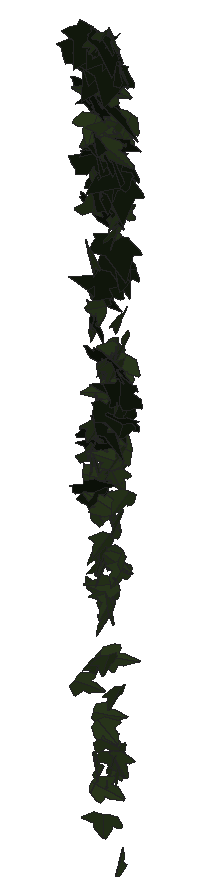
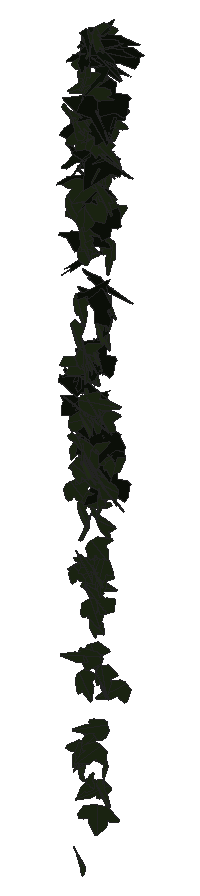
# SketchUp Ruby script. Lengths in inches.
U = 1.inch
M = Sketchup.active_model
def pt(a) = Geom::Point3d.new(a.map { |v| v * U })
def face(e, loops, mat)
  f = e.add_face(loops[0].map { |a| pt(a) })
  loops[1..].each { |l| e.add_face(l.map { |a| pt(a) }).erase! }
  f.material = f.back_material = mat if mat
  f
end
# faces: each face lists its corners as indices into pts; further lists are holes
def faces(e, pts, list, mat = nil) = list.each { |f| face(e, (f[0].is_a?(Array) ? f : [f]).map { |l| l.map { |i| pts[i] } }, mat) }
# xy, xz, yz: faces in a plane at the given z, y or x. An outline is a flat list of corners, or four numbers for a rectangle; further outlines are holes
def ring(l) = l.size == 4 ? [[l[0], l[1]], [l[2], l[1]], [l[2], l[3]], [l[0], l[3]]] : l.each_slice(2).to_a
def flat(e, list, mat, &to3) = list.each { |f| face(e, (f[0].is_a?(Array) ? f : [f]).map { |l| ring(l).map { |u, v| to3.(u, v) } }, mat) }
def xy(e, z, list, mat = nil) = flat(e, list, mat) { |x, y| [x, y, z] }
def xz(e, y, list, mat = nil) = flat(e, list, mat) { |x, z| [x, y, z] }
def yz(e, x, list, mat = nil) = flat(e, list, mat) { |y, z| [x, y, z] }
def lines(e, pts, list) = list.each { |a, b| e.add_line(pt(pts[a]), pt(pts[b])) }
# prism: a flat outline (further loops are holes) pulled along v
def prism(e, loops, v, mat = nil)
  f = face(e, loops, mat); d = Geom::Vector3d.new(v.map { |x| x * U })
  f.pushpull(f.normal.samedirection?(d) ? d.length : -d.length)
end
def box(e, o, s, mat = nil) = prism(e, [[o, [o[0] + s[0], o[1], o[2]], [o[0] + s[0], o[1] + s[1], o[2]], [o[0], o[1] + s[1], o[2]]]], [0, 0, s[2]], mat)
def at(x, y, z, deg = 0) = Geom::Transformation.translation(pt([x, y, z])) * Geom::Transformation.rotation(ORIGIN, Z_AXIS, deg.degrees)
def axes(o, x, y, z) = Geom::Transformation.new([*x, 0, *y, 0, *z, 0, *pt(o).to_a, 1])
def part(name) = M.definitions.add(name)
# library, detail: a bought-in or finely detailed component or shape, given as its bounding box
def library(name, o, s) = part(name).tap { |d| box(d.entities, o, s) }
def detail(e, o, s) = box(e.add_group.entities, o, s)
def put(e, d, t, mat = nil) = e.add_instance(d, t).tap { |i| i.material = mat if mat }
def group(e, t, mat = nil) = e.add_group.tap { |g| g.transformation = t; g.material = mat if mat }.entities
root = M.entities
M.materials.add("1026 AP 7946 SUNNY SIDE UP").color = [254, 231, 186]
M.materials.add("efeu1").color = [18, 25, 13]
M.materials.add("efeu2").color = [43, 57, 29]
c1 = part("ivyleaf_10")
p = [[0,0.5,-0.03],[-0.0625,2.02,-0.43],[-0.19,2.01,-0.46],[-0.54,1.05,-0.29],[-0.52,0.625,-0.18],[-0.83,0.76,-0.28],
  [-1.16,0.64,-0.33],[-1.15,0.33,-0.24],[-0.77,-0.39,0.02],[-0.3,-0.51,0.16],[0.04,-0.48,0.23],[-0.02,2.01,-0.4375],
  [-0.06,2.01,-0.43],[0.04,-0.49,0.23],[0.67,-0.49,0.14],[1.38,0.36,-0.2],[1.375,0.51,-0.24],[0.81,0.65,-0.19],
  [0.62,0.59,-0.15],[0.6,1.09,-0.28],[0.5,1.23,-0.31]]
faces(c1.entities,p,[[0,1,2,3,4,5,6,7,8,9,10],[11,12,0,13,14,15,16,17,18,19,20]],"efeu2")
c2 = part("ivyleaf_9")
p = [[1.54,2.16,1.25],[1.36,2.04,1.19],[-0.21,0.99,0.68],[-0.71,1.11,0.82],[-0.85,0.86,0.67],[-0.8,0.17,0.21],
  [-0.9,-0.01,0.1],[-0.67,-0.16,-0.02],[-0.08,-0.08,-0.05],[-0.03,-0.6,-0.4],[0.65,-0.88,-0.66],[0.83,-0.6,-0.49],
  [1.29,-0.42,-0.43],[1.8125,-0.07,-0.26],[1.21,0.44,0.15]]
faces(c2.entities,p,[[0,1,2,3,4,5,6,7,8,9,10,11,12,13,14]],"efeu1")
put(root,c1,axes([99.76,212.49,266.375],[0.08517,0.006,-0.24182],[-0.3837,0.00239,-0.05363],[0.00175,0.23145,0.01006]),"1026 AP 7946 SUNNY SIDE UP")
put(root,c2,axes([99.56,212.48,266.26],[0.11075,0.21792,-0.06124],[-0.02401,-0.05844,-0.24433],[-0.38297,0.06669,-0.00239]),"1026 AP 7946 SUNNY SIDE UP")
put(root,c1,axes([99.72,212.47,265.36],[-0.24212,0.01726,0.18054],[-0.27936,-0.06579,-0.14291],[0.06741,-0.21066,0.05618]),"1026 AP 7946 SUNNY SIDE UP")
put(root,c1,axes([99.48,212.33,258.37],[-0.13846,-0.2022,-0.00145],[-0.01239,0.00432,0.23331],[-0.34303,0.08146,-0.00784]),"1026 AP 7946 SUNNY SIDE UP")
put(root,c1,axes([99.56,212.56,264.48],[0.26352,-0.15611,-0.06063],[-0.07644,0.03216,-0.23505],[0.27014,0.16139,-0.00736]),"1026 AP 7946 SUNNY SIDE UP")
put(root,c2,axes([99.64,212.18,264.87],[-0.35667,0.10368,-0.02563],[-0.02399,0.02832,0.2504],[0.17957,0.20972,-0.01745]),"1026 AP 7946 SUNNY SIDE UP")
put(root,c1,axes([99.71,212.37,257.11],[0.16693,-0.00017,0.20356],[-0.29635,0.06729,0.10477],[-0.09333,-0.21398,0.03141]),"1026 AP 7946 SUNNY SIDE UP")
put(root,c1,axes([99.48,212.51,265.76],[0.28202,-0.15147,0.04086],[-0.02126,0.04548,0.23985],[-0.26515,-0.16475,0.02422]),"1026 AP 7946 SUNNY SIDE UP")
put(root,c1,axes([99.54,212.5625,253.86],[0.16321,-0.18368,0.02591],[0.0078,-0.02725,-0.21731],[0.29164,0.10352,-0.00869]),"1026 AP 7946 SUNNY SIDE UP")
put(root,c1,axes([99.53,212.38,263.85],[-0.18724,-0.24297,-0.03657],[-0.02415,-0.03047,0.27857],[-0.38504,0.12007,0.00031]),"1026 AP 7946 SUNNY SIDE UP")
put(root,c2,axes([99.78,212.16,257.77],[-0.28086,0.06421,-0.18603],[-0.25595,0.08041,0.19541],[0.16009,0.2412,-0.01395]),"1026 AP 7946 SUNNY SIDE UP")
put(root,c1,axes([99.53,212.47,256.28],[-0.02105,-0.17932,-0.11094],[0.06019,0.10297,-0.18267],[0.32252,-0.03092,0.02685]),"1026 AP 7946 SUNNY SIDE UP")
put(root,c2,axes([99.37,212.375,266.55],[0.42706,0.06153,-0.00314],[0.00359,-0.0254,-0.28585],[-0.09683,0.27043,-0.02446]),"1026 AP 7946 SUNNY SIDE UP")
put(root,c1,axes([99.41,212.1,253.51],[-0.09836,-0.09431,-0.18432],[0.22061,0.11389,-0.11205],[0.22802,-0.15087,0.0289]),"1026 AP 7946 SUNNY SIDE UP")
put(root,c2,axes([99.6,212.3125,267.66],[-0.3275,-0.14109,-0.01632],[0.03935,-0.00907,-0.25502],[0.23734,-0.19318,0.01976]),"1026 AP 7946 SUNNY SIDE UP")
put(root,c1,axes([99.44,212.47,258.59],[-0.21275,0.07912,-0.11622],[0.14396,-0.07034,-0.15918],[-0.17866,-0.15089,0.01012]),"1026 AP 7946 SUNNY SIDE UP")
put(root,c1,axes([99.58,212.42,253.91],[-0.03475,-0.21835,-0.02189],[0.00904,0.01953,-0.22594],[0.34465,-0.02253,0.00372]),"1026 AP 7946 SUNNY SIDE UP")
put(root,c1,axes([99.625,212.14,263.01],[-0.26211,0.17039,0.07833],[-0.10034,0.04237,-0.24482],[-0.27504,-0.17784,0.01467]),"1026 AP 7946 SUNNY SIDE UP")
put(root,c2,axes([99.36,212.2,267.45],[-0.07303,-0.10387,-0.24371],[0.1798,0.20019,-0.11714],[0.38252,-0.11393,0.00853]),"1026 AP 7946 SUNNY SIDE UP")
put(root,c1,axes([99.69,212.1,261.41],[0.08371,-0.05213,0.26704],[-0.23495,0.21258,0.07681],[-0.34355,-0.15808,0.01254]),"1026 AP 7946 SUNNY SIDE UP")
put(root,c1,axes([99.55,212.52,251.41],[0.15767,-0.17338,0.07724],[0.0386,-0.07332,-0.20623],[0.29513,0.10222,-0.01429]),"1026 AP 7946 SUNNY SIDE UP")
put(root,c1,axes([99.58,212.625,258.77],[-0.01506,-0.15587,0.15875],[0.03486,-0.15503,-0.16011],[0.34386,0.00889,0.02318]),"1026 AP 7946 SUNNY SIDE UP")
put(root,c2,axes([99.36,212.59,265.85],[0.21526,-0.15628,0.09252],[0.08295,-0.07417,-0.21632],[0.29333,0.13566,-0.00672]),"1026 AP 7946 SUNNY SIDE UP")
put(root,c1,axes([99.8,212.61,259.78],[-0.06157,0.02381,0.22766],[-0.2122,-0.18068,-0.00564],[0.27744,-0.13291,0.04621]),"1026 AP 7946 SUNNY SIDE UP")
put(root,c2,axes([99.35,212.51,263.73],[0.32534,-0.07202,-0.12624],[0.20214,0.00416,0.22186],[-0.09403,-0.24023,0.04016]),"1026 AP 7946 SUNNY SIDE UP")
put(root,c1,axes([99.47,212.37,258.27],[-0.04813,0.0255,0.22754],[0.22348,-0.16655,0.03794],[0.28582,0.13452,0.00866]),"1026 AP 7946 SUNNY SIDE UP")
put(root,c1,axes([99.64,212.45,257.75],[0.05416,-0.15376,-0.15025],[0.00352,0.14021,-0.16437],[0.35109,0.02231,0.02483]),"1026 AP 7946 SUNNY SIDE UP")
put(root,c1,axes([99.64,212.4375,256.05],[-0.04484,-0.20123,-0.04817],[0.01543,0.04467,-0.20909],[0.32407,-0.02997,0.00329]),"1026 AP 7946 SUNNY SIDE UP")
put(root,c2,axes([99.6,212.29,259.03],[0.21165,0.18417,-0.00479],[0.01282,-0.0134,-0.23784],[-0.3126,0.12415,-0.01299]),"1026 AP 7946 SUNNY SIDE UP")
put(root,c1,axes([99.64,212.43,261.38],[0.09194,-0.21347,0.04998],[0.00429,-0.05076,-0.22806],[0.34462,0.05758,-0.0105]),"1026 AP 7946 SUNNY SIDE UP")
put(root,c1,axes([99.6,212.3,265.82],[0.35179,0.08539,-0.03383],[-0.03769,-0.03161,-0.23939],[-0.15058,0.20741,-0.01911]),"1026 AP 7946 SUNNY SIDE UP")
put(root,c1,axes([99.58,212.41,259.63],[-0.07566,0.14133,-0.10499],[0.0339,-0.09828,-0.15975],[-0.29185,-0.04805,0.00866]),"1026 AP 7946 SUNNY SIDE UP")
put(root,c2,axes([99.73,212.31,258.75],[0.17736,0.15221,-0.12069],[-0.13961,-0.08201,-0.19783],[-0.29187,0.13172,0.02129]),"1026 AP 7946 SUNNY SIDE UP")
put(root,c1,axes([99.58,212.59,256.1875],[0.12198,-0.14491,0.14792],[0.10082,-0.12944,-0.17005],[0.30547,0.10059,-0.00294]),"1026 AP 7946 SUNNY SIDE UP")
put(root,c1,axes([99.77,212.29,264.79],[-0.33099,0.02229,0.07366],[-0.11999,-0.02094,-0.20837],[-0.02367,-0.20561,0.02628]),"1026 AP 7946 SUNNY SIDE UP")
put(root,c2,axes([99.59,212.38,265.09],[0.26162,0.1795,0.00575],[0.02563,-0.0089,-0.25151],[-0.28117,0.1662,-0.01757]),"1026 AP 7946 SUNNY SIDE UP")
put(root,c2,axes([99.93,212.28,262.27],[-0.22067,0.10407,0.14173],[-0.19513,0.06503,-0.17648],[-0.20641,-0.17274,0.01532]),"1026 AP 7946 SUNNY SIDE UP")
put(root,c1,axes([99.64,212.24,258.48],[-0.17778,0.20569,0.00456],[-0.01956,-0.00312,-0.24149],[-0.32288,-0.11307,0.01212]),"1026 AP 7946 SUNNY SIDE UP")
put(root,c2,axes([99.62,212.35,267.4],[-0.26915,-0.16923,-0.05648],[0.11001,0.00745,-0.24421],[0.27891,-0.16625,0.04182]),"1026 AP 7946 SUNNY SIDE UP")
put(root,c2,axes([99.57,212.37,267.01],[0.26014,-0.10943,-0.15047],[-0.17492,0.09447,-0.19974],[0.24431,0.18416,0.01721]),"1026 AP 7946 SUNNY SIDE UP")
put(root,c2,axes([99.6,212.4,261.31],[-0.08483,-0.02212,0.25567],[-0.03003,-0.25293,-0.02897],[0.39082,-0.02424,0.05327]),"1026 AP 7946 SUNNY SIDE UP")
put(root,c1,axes([99.66,212.26,258.9],[0.17579,-0.19766,0.04183],[0.02888,-0.0381,-0.23941],[0.34169,0.10491,-0.00128]),"1026 AP 7946 SUNNY SIDE UP")
put(root,c1,axes([99.54,212.47,255.36],[-0.25359,0.00555,0.13479],[0.20485,0.02747,0.16443],[-0.02049,0.20583,-0.02435]),"1026 AP 7946 SUNNY SIDE UP")
put(root,c1,axes([99.61,212.31,251.8],[-0.10505,0.14077,-0.13681],[0.05466,-0.13033,-0.16014],[-0.30023,-0.07298,0.01871]),"1026 AP 7946 SUNNY SIDE UP")
put(root,c1,axes([99.63,212.32,264.64],[-0.14063,0.19537,-0.05433],[0.02319,-0.05206,-0.22777],[-0.34299,-0.08362,0.00688]),"1026 AP 7946 SUNNY SIDE UP")
put(root,c2,axes([99.39,212.58,261.93],[0.17479,-0.06802,-0.21867],[0.34796,0.00888,0.11672],[-0.03681,-0.2391,0.06503]),"1026 AP 7946 SUNNY SIDE UP")
put(root,c1,axes([99.75,212.54,255.37],[-0.14437,-0.18315,0.04186],[-0.0119,-0.04275,-0.21094],[0.2951,-0.09132,0.01197]),"1026 AP 7946 SUNNY SIDE UP")
put(root,c2,axes([99.68,212.52,267.43],[-0.21776,-0.18332,0.12187],[0.01993,-0.14774,-0.2195],[0.34337,-0.10768,0.09003]),"1026 AP 7946 SUNNY SIDE UP")
put(root,c1,axes([99.67,212.49,264.6],[-0.05944,0.13981,0.19187],[0.0932,-0.16886,0.15173],[0.37192,0.06466,-0.00736]),"1026 AP 7946 SUNNY SIDE UP")
put(root,c1,axes([99.75,212.45,256.63],[-0.08791,-0.16824,0.11127],[-0.00764,-0.11195,-0.1813],[0.31509,-0.04966,0.02665]),"1026 AP 7946 SUNNY SIDE UP")
put(root,c1,axes([99.73,212.31,267.68],[-0.01453,-0.25488,0.06221],[0.03014,-0.06188,-0.27311],[0.44404,-0.00414,0.02057]),"1026 AP 7946 SUNNY SIDE UP")
put(root,c1,axes([99.77,212.22,259.29],[-0.07295,-0.21505,0.06073],[-0.02556,-0.05769,-0.23556],[0.37792,-0.04541,-0.00421]),"1026 AP 7946 SUNNY SIDE UP")
put(root,c2,axes([99.89,212.3,267.56],[-0.1829,0.2258,-0.07515],[0.03671,-0.07065,-0.2686],[-0.40124,-0.10939,0.00968]),"1026 AP 7946 SUNNY SIDE UP")
put(root,c2,axes([99.6,212.03,257.92],[0.29133,0.14779,0.05738],[0.08372,0.02102,-0.24345],[-0.23332,0.19208,-0.01571]),"1026 AP 7946 SUNNY SIDE UP")
put(root,c1,axes([99.87,212.13,261.91],[0.15458,-0.12495,-0.15872],[-0.17639,0.10471,-0.16315],[0.27537,0.13721,-0.01541]),"1026 AP 7946 SUNNY SIDE UP")
put(root,c1,axes([99.45,212.39,257.93],[0.05124,-0.04101,-0.22691],[0.34489,-0.03838,0.04061],[-0.07002,-0.21909,0.03399]),"1026 AP 7946 SUNNY SIDE UP")
put(root,c2,axes([99.68,212.57,265.57],[-0.12461,-0.20667,0.12007],[0.02266,-0.12803,-0.2223],[0.3733,-0.06122,0.05357]),"1026 AP 7946 SUNNY SIDE UP")
put(root,c2,axes([99.9,212.46,262.01],[-0.2271,-0.15455,0.07391],[0.06496,0.06073,0.21941],[-0.28136,0.13877,-0.009]),"1026 AP 7946 SUNNY SIDE UP")
put(root,c2,axes([99.82,212.3125,267.08],[-0.39642,-0.08295,-0.07372],[0.13419,-0.02374,-0.26081],[0.12272,-0.242,0.04705]),"1026 AP 7946 SUNNY SIDE UP")
put(root,c1,axes([99.95,212.37,255.72],[0.08255,0.00781,-0.18142],[-0.26703,-0.06419,-0.05236],[-0.10825,0.1643,-0.00919]),"1026 AP 7946 SUNNY SIDE UP")
put(root,c1,axes([99.84,212.4,265.62],[-0.37722,0.02843,0.02257],[-0.03972,-0.02052,-0.23883],[-0.0446,-0.22223,0.02176]),"1026 AP 7946 SUNNY SIDE UP")
put(root,c2,axes([99.58,212.3,266.19],[0.0511,-0.05451,0.22063],[0.11242,-0.19619,-0.06843],[0.34519,0.07196,-0.01038]),"1026 AP 7946 SUNNY SIDE UP")
put(root,c1,axes([99.61,212.45,252.75],[-0.01876,-0.05913,-0.20108],[0.25356,0.11643,-0.04589],[0.19549,-0.15669,0.04023]),"1026 AP 7946 SUNNY SIDE UP")
put(root,c1,axes([99.78,212.45,254.95],[0.03551,-0.1566,0.1309],[0.05105,-0.12427,-0.16332],[0.31385,0.03793,0.01175]),"1026 AP 7946 SUNNY SIDE UP")
put(root,c1,axes([99.65,212.44,258.03],[0.21028,-0.15537,-0.09212],[0.11823,-0.05146,0.20973],[-0.25513,-0.15191,0.02126]),"1026 AP 7946 SUNNY SIDE UP")
put(root,c1,axes([99.75,212.35,259.56],[0.07645,0.21074,0.01436],[0.01157,0.00945,-0.23052],[-0.35801,0.04531,-0.00438]),"1026 AP 7946 SUNNY SIDE UP")
put(root,c1,axes([99.93,212.29,257.44],[0.08276,0.14413,0.1551],[-0.12307,-0.12501,0.15961],[0.32193,-0.08484,0.02114]),"1026 AP 7946 SUNNY SIDE UP")
put(root,c2,axes([99.65,212.29,260.72],[0.40283,-0.03703,-0.03931],[-0.06397,-0.01724,-0.26574],[0.05346,0.25841,-0.02182]),"1026 AP 7946 SUNNY SIDE UP")
put(root,c2,axes([99.76,212.54,264.97],[-0.12989,-0.15559,0.1382],[0.02286,-0.14365,-0.17608],[0.34464,-0.04911,0.06377]),"1026 AP 7946 SUNNY SIDE UP")
put(root,c1,axes([99.72,212.44,252.19],[-0.12025,-0.10156,-0.16408],[0.18086,0.11048,-0.1293],[0.23464,-0.13721,0.01557]),"1026 AP 7946 SUNNY SIDE UP")
put(root,c1,axes([99.84,212.69,263.07],[-0.01368,-0.06503,0.18943],[0.02121,-0.17775,-0.07148],[0.32067,0.00898,0.01281]),"1026 AP 7946 SUNNY SIDE UP")
put(root,c1,axes([99.8125,212.625,251.52],[0.03859,0.1436,-0.14529],[-0.03627,-0.13996,-0.1509],[-0.31531,0.03367,-0.00043]),"1026 AP 7946 SUNNY SIDE UP")
put(root,c1,axes([99.94,212.43,265.73],[-0.18153,-0.23042,0.11146],[-0.05352,-0.10521,-0.26565],[0.39756,-0.11938,0.01513]),"1026 AP 7946 SUNNY SIDE UP")
put(root,c1,axes([99.73,212.375,252.54],[0.11135,0.16358,0.10443],[0.0773,0.08803,-0.18289],[-0.29176,0.08575,-0.0086]),"1026 AP 7946 SUNNY SIDE UP")
put(root,c1,axes([99.8,212.55,259.82],[0.20376,-0.16987,0.10496],[0.06773,-0.09585,-0.21954],[0.30481,0.13485,-0.02138]),"1026 AP 7946 SUNNY SIDE UP")
put(root,c1,axes([99.88,212.35,260.58],[0.02751,-0.21013,-0.07622],[-0.00665,0.07269,-0.21679],[0.34961,0.01791,0.00188]),"1026 AP 7946 SUNNY SIDE UP")
put(root,c1,axes([99.72,212.33,260.49],[0.08061,-0.14579,-0.17154],[0.09898,-0.14736,0.16193],[-0.3517,-0.07489,0.00625]),"1026 AP 7946 SUNNY SIDE UP")
put(root,c1,axes([99.82,212.55,267.6],[-0.19849,0.20156,-0.03869],[0.0148,-0.03969,-0.24967],[-0.34811,-0.11661,0.01144]),"1026 AP 7946 SUNNY SIDE UP")
put(root,c1,axes([100.03,212.38,258.46],[0.04142,0.05556,0.19093],[-0.20648,-0.13083,0.05987],[0.23912,-0.12259,0.01863]),"1026 AP 7946 SUNNY SIDE UP")
put(root,c1,axes([99.89,212.59,263.39],[0.03421,-0.23632,-0.01199],[0.0049,0.01062,-0.24439],[0.37192,0.0216,0.00432]),"1026 AP 7946 SUNNY SIDE UP")
put(root,c1,axes([99.82,212.26,256.11],[0.13671,-0.13485,0.09886],[0.06761,-0.08566,-0.16912],[0.27083,0.08946,-0.00768]),"1026 AP 7946 SUNNY SIDE UP")
put(root,c2,axes([99.76,212.44,264.53],[-0.21683,-0.08931,-0.16028],[0.28374,-0.01465,-0.14465],[0.07785,-0.19536,0.0808]),"1026 AP 7946 SUNNY SIDE UP")
put(root,c1,axes([99.84,212.66,259.44],[0.1465,-0.18838,0.11483],[0.07313,-0.10252,-0.21708],[0.3372,0.10408,-0.00281]),"1026 AP 7946 SUNNY SIDE UP")
put(root,c2,axes([99.76,212.35,264.25],[0.13297,-0.18296,-0.11837],[-0.07962,0.09758,-0.21166],[0.35192,0.0912,-0.00316]),"1026 AP 7946 SUNNY SIDE UP")
put(root,c1,axes([99.69,212.375,266.68],[-0.18696,-0.08802,-0.20535],[0.3045,0.07252,-0.14575],[0.18536,-0.2079,0.03232]),"1026 AP 7946 SUNNY SIDE UP")
put(root,c1,axes([99.86,212.43,255.28],[-0.0589,-0.1071,0.17561],[0.08463,-0.173,-0.10044],[0.30587,0.02724,0.06161]),"1026 AP 7946 SUNNY SIDE UP")
put(root,c1,axes([99.92,212.48,260.67],[0.03124,-0.19848,-0.12058],[0.00434,0.11655,-0.20441],[0.36139,0.01576,0.01288]),"1026 AP 7946 SUNNY SIDE UP")
put(root,c1,axes([99.94,212.17,250.66],[-0.30878,-0.10361,0.01073],[-0.00117,-0.02207,-0.22801],[0.16383,-0.19544,0.01859]),"1026 AP 7946 SUNNY SIDE UP")
put(root,c1,axes([99.75,212.25,251.27],[0.07133,0.11717,0.18855],[0.13184,0.16232,-0.12798],[-0.31429,0.09468,-0.0109]),"1026 AP 7946 SUNNY SIDE UP")
put(root,c1,axes([99.88,212.52,265.47],[-0.31204,-0.15732,-0.01699],[0.09922,-0.04807,-0.24714],[0.24905,-0.17796,0.07717]),"1026 AP 7946 SUNNY SIDE UP")
put(root,c1,axes([99.92,212.54,260.79],[-0.10308,-0.16356,0.1647],[0.04362,-0.17166,-0.16923],[0.358,-0.02618,0.06804]),"1026 AP 7946 SUNNY SIDE UP")
put(root,c1,axes([99.79,212.64,260.83],[0.22195,-0.11585,0.14341],[0.15193,-0.1021,-0.18817],[0.24181,0.17048,-0.01341]),"1026 AP 7946 SUNNY SIDE UP")
put(root,c1,axes([99.96,212.5625,260.43],[0.28205,0.06814,-0.10059],[-0.13336,-0.05684,-0.19184],[-0.14669,0.18268,-0.01901]),"1026 AP 7946 SUNNY SIDE UP")
put(root,c1,axes([99.97,212.5625,256.3],[0.23664,-0.14088,-0.04868],[-0.06491,0.02379,-0.21195],[0.22404,0.15569,-0.00998]),"1026 AP 7946 SUNNY SIDE UP")
put(root,c1,axes([99.83,212.375,255.32],[-0.15243,0.13076,-0.13596],[0.09538,-0.11931,-0.16744],[-0.277,-0.11304,0.01716]),"1026 AP 7946 SUNNY SIDE UP")
put(root,c2,axes([99.82,212.69,267.18],[-0.01422,-0.02864,0.2331],[0.00994,-0.21821,-0.03348],[0.37329,0.00472,0.00977]),"1026 AP 7946 SUNNY SIDE UP")
put(root,c1,axes([99.9375,212.58,256.84],[-0.12702,0.15911,0.1054],[0.05997,-0.09426,0.18311],[0.29054,0.08901,0.00828]),"1026 AP 7946 SUNNY SIDE UP")
put(root,c1,axes([99.97,212.43,258.32],[0.08131,-0.20026,0.04766],[-0.00252,-0.04872,-0.22071],[0.34922,0.04628,-0.01269]),"1026 AP 7946 SUNNY SIDE UP")
put(root,c1,axes([99.99,212.22,254.18],[-0.08911,-0.19916,0.01559],[0.00146,-0.01717,-0.21334],[0.31419,-0.05641,0.00541]),"1026 AP 7946 SUNNY SIDE UP")
put(root,c1,axes([100.01,212.47,267.03],[-0.29611,0.17317,0.05292],[-0.08462,0.01645,-0.26176],[-0.29269,-0.17995,0.02214]),"1026 AP 7946 SUNNY SIDE UP")
put(root,c1,axes([99.79,212.5,256.2],[-0.17725,-0.0322,-0.15186],[0.24407,0.00003,-0.11365],[0.0325,-0.1758,0.02526]),"1026 AP 7946 SUNNY SIDE UP")
put(root,c2,axes([99.97,212.34,265.48],[0.25384,0.15053,-0.08462],[-0.08124,-0.06645,-0.22771],[-0.27857,0.15654,-0.0107]),"1026 AP 7946 SUNNY SIDE UP")
put(root,c1,axes([99.99,212.49,263.86],[-0.29025,-0.13467,-0.00602],[0.02407,-0.01177,-0.23237],[0.22743,-0.17062,0.01691]),"1026 AP 7946 SUNNY SIDE UP")
put(root,c2,axes([99.9,212.37,265.15],[0.20192,-0.12472,-0.15083],[-0.16048,0.10227,-0.18307],[0.27378,0.15193,0.00393]),"1026 AP 7946 SUNNY SIDE UP")
put(root,c1,axes([99.97,212.6,258.875],[0.32134,-0.06225,-0.00991],[-0.02266,-0.01365,-0.21274],[0.1042,0.18899,-0.01569]),"1026 AP 7946 SUNNY SIDE UP")
put(root,c2,axes([99.83,212.34,267.58],[0.00157,-0.22997,0.12597],[0.06068,-0.12209,-0.2351],[0.406,0.01914,0.03465]),"1026 AP 7946 SUNNY SIDE UP")
put(root,c1,axes([99.98,212.47,258.42],[0.18401,-0.17102,0.04573],[0.03041,-0.04182,-0.21722],[0.29862,0.10964,-0.00606]),"1026 AP 7946 SUNNY SIDE UP")
put(root,c1,axes([100.05,212.41,258.74],[-0.12518,0.14743,0.10092],[-0.10497,0.07153,-0.17413],[-0.27601,-0.09406,0.02045]),"1026 AP 7946 SUNNY SIDE UP")
put(root,c2,axes([99.81,212.45,260.57],[0.33179,-0.08097,0.00205],[-0.00773,-0.01871,-0.22584],[0.13732,0.19458,-0.01766]),"1026 AP 7946 SUNNY SIDE UP")
put(root,c1,axes([100.07,212.57,260.61],[0.28846,0.09102,-0.11709],[-0.13945,-0.07619,-0.20982],[-0.18239,0.20221,-0.02476]),"1026 AP 7946 SUNNY SIDE UP")
put(root,c1,axes([99.96,212.48,264.36],[-0.29848,-0.08758,-0.09343],[0.16175,-0.00234,-0.20574],[0.13159,-0.19578,0.04098]),"1026 AP 7946 SUNNY SIDE UP")
put(root,c2,axes([99.86,212.23,259.31],[0.14957,-0.2089,-0.02063],[-0.00786,0.01601,-0.24249],[0.35564,0.08821,0.00332]),"1026 AP 7946 SUNNY SIDE UP")
put(root,c1,axes([100.07,212.58,256.03],[-0.11674,-0.14125,0.12949],[0.0128,-0.1381,-0.15474],[0.29787,-0.04942,0.0574]),"1026 AP 7946 SUNNY SIDE UP")
put(root,c1,axes([100.09,212.33,260.62],[-0.0658,-0.2194,0.03896],[-0.00671,-0.03895,-0.2303],[0.35034,-0.04195,0.0029]),"1026 AP 7946 SUNNY SIDE UP")
put(root,c1,axes([100.06,212.59,258.28],[0.02544,-0.15704,0.14511],[0.02287,-0.141,-0.16347],[0.33186,0.02176,0.00014]),"1026 AP 7946 SUNNY SIDE UP")
put(root,c2,axes([100.02,212.3125,267.13],[-0.20496,-0.22709,-0.00198],[0.01526,-0.00603,-0.27519],[0.38519,-0.12059,0.00985]),"1026 AP 7946 SUNNY SIDE UP")
put(root,c2,axes([100.2,212.25,259.49],[0.12096,0.15268,-0.15322],[-0.15214,-0.11665,-0.18015],[-0.32358,0.11192,0.02742]),"1026 AP 7946 SUNNY SIDE UP")
put(root,c2,axes([99.93,212.52,262.83],[0.03031,-0.24231,-0.04878],[0.01096,0.04663,-0.24991],[0.38765,0.01762,0.01088]),"1026 AP 7946 SUNNY SIDE UP")
put(root,c1,axes([100.14,212.22,259.68],[0.07353,-0.19155,-0.13689],[-0.05037,0.12182,-0.20854],[0.38534,0.05247,-0.00114]),"1026 AP 7946 SUNNY SIDE UP")
put(root,c2,axes([100.23,212.28,264.9375],[-0.39948,-0.00371,-0.01979],[0.03175,-0.02215,-0.25114],[0.00332,-0.23501,0.02068]),"1026 AP 7946 SUNNY SIDE UP")
put(root,c2,axes([99.81,212.47,266.16],[0.15213,-0.21367,0.0967],[0.13172,-0.06671,-0.24479],[0.37309,0.11068,0.04699]),"1026 AP 7946 SUNNY SIDE UP")
put(root,c1,axes([100.05,212.33,258.2],[-0.2286,-0.11629,-0.06709],[0.09793,0.02634,-0.18926],[0.20038,-0.14553,0.01596]),"1026 AP 7946 SUNNY SIDE UP")
put(root,c2,axes([99.96,212.26,259.6875],[0.03996,-0.20252,-0.11215],[-0.01636,0.10168,-0.21684],[0.38466,0.02537,0.00243]),"1026 AP 7946 SUNNY SIDE UP")
put(root,c2,axes([100.12,212.375,259.92],[-0.00156,0.04896,0.22111],[-0.18305,-0.17727,0.04214],[0.30913,-0.10472,0.02607]),"1026 AP 7946 SUNNY SIDE UP")
put(root,c1,axes([99.88,212.375,254.12],[0.00519,-0.0473,-0.21244],[0.30602,0.08091,-0.01546],[0.12942,-0.18942,0.04507]),"1026 AP 7946 SUNNY SIDE UP")
put(root,c2,axes([100.39,212.43,260.04],[-0.10812,-0.01485,-0.21444],[-0.30362,-0.09097,0.0669],[-0.1544,0.18927,0.0186]),"1026 AP 7946 SUNNY SIDE UP")
put(root,c1,axes([100.11,212.41,252.05],[-0.01111,-0.1643,-0.13991],[0.04737,0.13281,-0.16753],[0.33088,-0.02453,0.01929]),"1026 AP 7946 SUNNY SIDE UP")
put(root,c1,axes([100.15,212.36,249.51],[0.18544,-0.12552,0.1252],[-0.10705,0.10295,0.17716],[-0.25386,-0.1351,0.01675]),"1026 AP 7946 SUNNY SIDE UP")
put(root,c1,axes([100.07,212.27,252.03],[-0.30696,-0.07649,-0.08262],[0.12834,0.00936,-0.21499],[0.11714,-0.21067,0.01905]),"1026 AP 7946 SUNNY SIDE UP")
put(root,c1,axes([100.12,212.41,257.27],[0.11116,-0.19208,0.05602],[0.02592,-0.05304,-0.21115],[0.3133,0.07254,-0.00241]),"1026 AP 7946 SUNNY SIDE UP")
put(root,c2,axes([100.05,212.6875,262.69],[-0.0627,-0.19183,0.10656],[-0.01948,-0.10163,-0.21042],[0.36833,-0.03803,0.00701]),"1026 AP 7946 SUNNY SIDE UP")
put(root,c1,axes([100.16,212.56,259.2],[-0.01149,0.01268,0.1975],[-0.00554,-0.18442,0.01088],[0.31358,-0.00279,0.00743]),"1026 AP 7946 SUNNY SIDE UP")
put(root,c2,axes([100.38,212.36,259.45],[-0.31309,0.11516,0.04714],[-0.08655,-0.00204,-0.23085],[-0.18958,-0.18927,0.02754]),"1026 AP 7946 SUNNY SIDE UP")
put(root,c2,axes([100.02,212.43,263.23],[-0.17895,-0.16833,-0.12787],[0.16565,0.07481,-0.20786],[0.30631,-0.13879,0.0377]),"1026 AP 7946 SUNNY SIDE UP")
put(root,c1,axes([100.18,212.29,253.51],[-0.02224,-0.21699,0.04859],[-0.00584,-0.04826,-0.2243],[0.34953,-0.01461,-0.00066]),"1026 AP 7946 SUNNY SIDE UP")
put(root,c1,axes([99.9,212.24,265.39],[-0.15953,0.00797,-0.22777],[0.33875,-0.07809,-0.09854],[-0.12648,-0.21919,0.02338]),"1026 AP 7946 SUNNY SIDE UP")
put(root,c2,axes([100.07,212.5,264.55],[-0.11534,-0.25369,-0.03808],[0.03107,0.03124,-0.27167],[0.40159,-0.07528,0.01008]),"1026 AP 7946 SUNNY SIDE UP")
put(root,c1,axes([100.21,212.44,258.67],[0.01152,0.1339,-0.17188],[-0.12229,-0.15109,-0.13879],[-0.33558,0.05965,0.04468]),"1026 AP 7946 SUNNY SIDE UP")
put(root,c1,axes([100.0625,212.5,251.72],[0.04643,-0.07659,0.20773],[0.1685,-0.17193,-0.08427],[0.29509,0.11023,0.01543]),"1026 AP 7946 SUNNY SIDE UP")
put(root,c2,axes([100.06,212.62,264.94],[-0.07602,-0.1884,0.15823],[0.04205,-0.16082,-0.19415],[0.38096,-0.01984,0.053]),"1026 AP 7946 SUNNY SIDE UP")
put(root,c1,axes([100.21,212.54,263.99],[0.00184,-0.19688,0.16248],[-0.01044,-0.1588,-0.20367],[0.39763,-0.00326,-0.0061]),"1026 AP 7946 SUNNY SIDE UP")
put(root,c1,axes([100.24,212.46,257.73],[-0.12976,-0.15969,0.11078],[-0.03025,-0.11055,-0.18343],[0.30201,-0.07968,0.02923]),"1026 AP 7946 SUNNY SIDE UP")
put(root,c1,axes([100.21,212.47,261.125],[0.12273,-0.24196,0.00008],[-0.0106,-0.0037,-0.26182],[0.38031,0.07798,-0.00732]),"1026 AP 7946 SUNNY SIDE UP")
put(root,c1,axes([100.15,212.61,265.91],[0.35331,-0.11983,0.01312],[0.00701,-0.02046,-0.25685],[0.20465,0.20758,-0.01385]),"1026 AP 7946 SUNNY SIDE UP")
put(root,c1,axes([100.22,212.35,261.73],[0.02937,-0.22901,-0.02314],[-0.006,0.02092,-0.23657],[0.36158,0.01895,-0.00205]),"1026 AP 7946 SUNNY SIDE UP")
